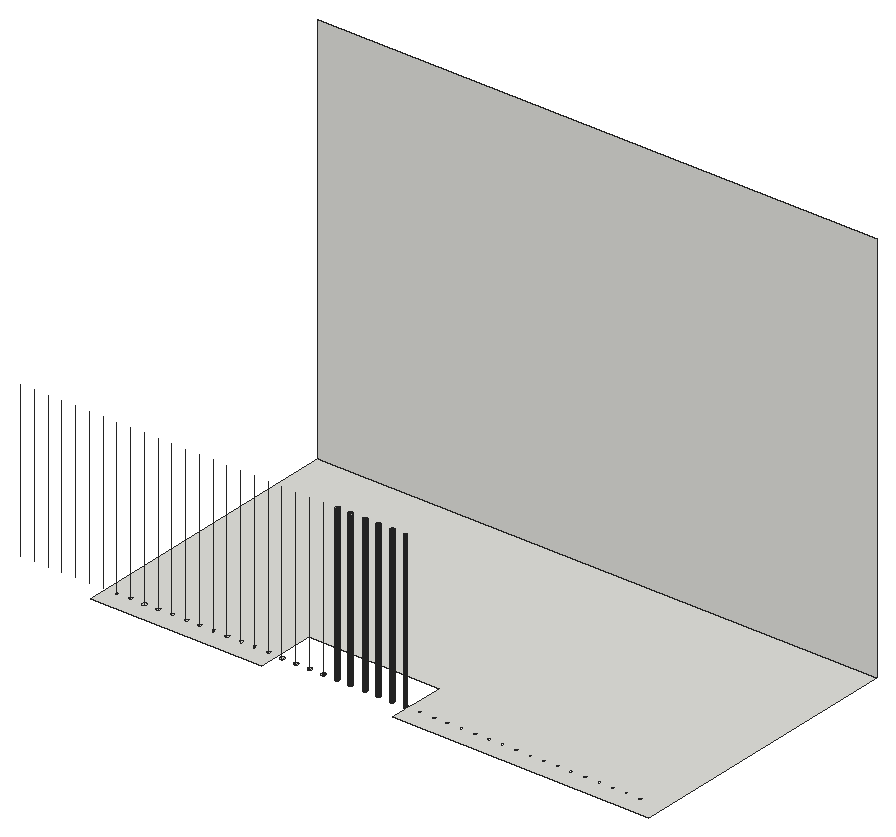
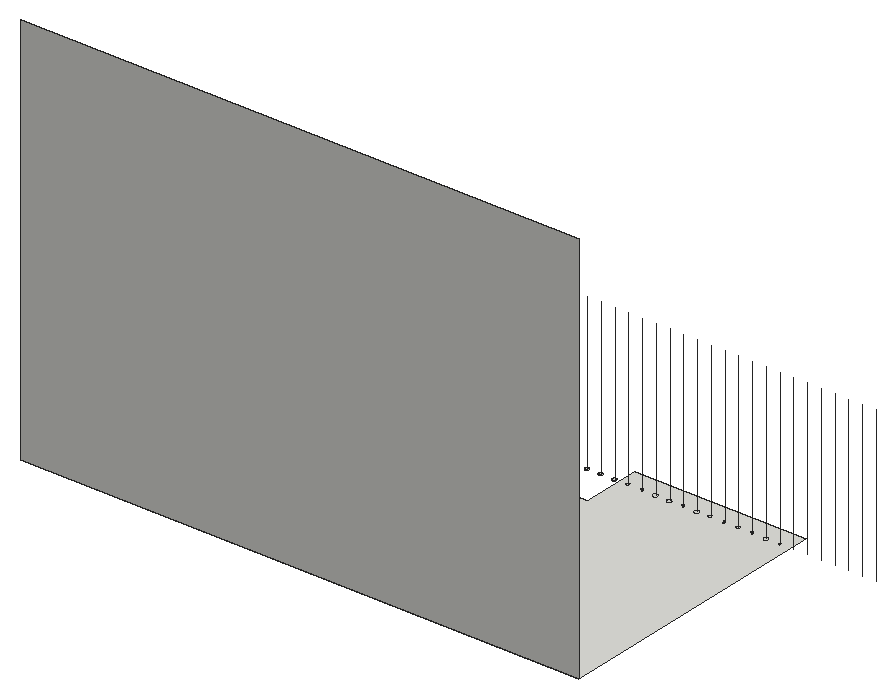
# SketchUp Ruby script. Lengths in inches.
U = 1.inch
M = Sketchup.active_model
def pt(a) = Geom::Point3d.new(a.map { |v| v * U })
def face(e, loops, mat)
  f = e.add_face(loops[0].map { |a| pt(a) })
  loops[1..].each { |l| e.add_face(l.map { |a| pt(a) }).erase! }
  f.material = f.back_material = mat if mat
  f
end
# faces: each face lists its corners as indices into pts; further lists are holes
def faces(e, pts, list, mat = nil) = list.each { |f| face(e, (f[0].is_a?(Array) ? f : [f]).map { |l| l.map { |i| pts[i] } }, mat) }
# xy, xz, yz: faces in a plane at the given z, y or x. An outline is a flat list of corners, or four numbers for a rectangle; further outlines are holes
def ring(l) = l.size == 4 ? [[l[0], l[1]], [l[2], l[1]], [l[2], l[3]], [l[0], l[3]]] : l.each_slice(2).to_a
def flat(e, list, mat, &to3) = list.each { |f| face(e, (f[0].is_a?(Array) ? f : [f]).map { |l| ring(l).map { |u, v| to3.(u, v) } }, mat) }
def xy(e, z, list, mat = nil) = flat(e, list, mat) { |x, y| [x, y, z] }
def xz(e, y, list, mat = nil) = flat(e, list, mat) { |x, z| [x, y, z] }
def yz(e, x, list, mat = nil) = flat(e, list, mat) { |y, z| [x, y, z] }
def lines(e, pts, list) = list.each { |a, b| e.add_line(pt(pts[a]), pt(pts[b])) }
# prism: a flat outline (further loops are holes) pulled along v
def prism(e, loops, v, mat = nil)
  f = face(e, loops, mat); d = Geom::Vector3d.new(v.map { |x| x * U })
  f.pushpull(f.normal.samedirection?(d) ? d.length : -d.length)
end
def box(e, o, s, mat = nil) = prism(e, [[o, [o[0] + s[0], o[1], o[2]], [o[0] + s[0], o[1] + s[1], o[2]], [o[0], o[1] + s[1], o[2]]]], [0, 0, s[2]], mat)
def at(x, y, z, deg = 0) = Geom::Transformation.translation(pt([x, y, z])) * Geom::Transformation.rotation(ORIGIN, Z_AXIS, deg.degrees)
def axes(o, x, y, z) = Geom::Transformation.new([*x, 0, *y, 0, *z, 0, *pt(o).to_a, 1])
def part(name) = M.definitions.add(name)
# library, detail: a bought-in or finely detailed component or shape, given as its bounding box
def library(name, o, s) = part(name).tap { |d| box(d.entities, o, s) }
def detail(e, o, s) = box(e.add_group.entities, o, s)
def put(e, d, t, mat = nil) = e.add_instance(d, t).tap { |i| i.material = mat if mat }
def group(e, t, mat = nil) = e.add_group.tap { |g| g.transformation = t; g.material = mat if mat }.entities
root = M.entities
xy(root,614.8125,[[[290.4375,124.5,363.4375,124.5,363.4375,149.5,419.5625,149.5,419.5625,124.5,528.75,124.5,528.75,246,290.4375,246],[300.98,132.01,300.77,132.04,300.58,132.125,300.41,132.25,300.28,132.42,300.2,132.62,300.17,132.83,300.2,133.04,300.28,133.23,300.41,133.4,300.58,133.53,300.77,133.61,300.98,133.64,301.19,133.61,301.39,133.53,301.56,133.4,301.6875,133.23,301.77,133.04,301.8,132.83,301.77,132.62,301.6875,132.42,301.56,132.25,301.39,132.125,301.19,132.04],[306.92,132.01,306.71,132.04,306.51,132.125,306.35,132.25,306.22,132.42,306.14,132.62,306.11,132.83,306.14,133.04,306.22,133.23,306.35,133.4,306.51,133.53,306.71,133.61,306.92,133.64,307.13,133.61,307.33,133.53,307.49,133.4,307.625,133.23,307.7,133.04,307.73,132.83,307.7,132.62,307.625,132.42,307.49,132.25,307.33,132.125,307.13,132.04],[312.8,132.01,312.58,132.04,312.39,132.125,312.22,132.25,312.09,132.42,312.01,132.62,311.98,132.83,312.01,133.04,312.09,133.23,312.22,133.4,312.39,133.53,312.58,133.61,312.8,133.64,313.01,133.61,313.2,133.53,313.37,133.4,313.5,133.23,313.58,133.04,313.61,132.83,313.58,132.62,313.5,132.42,313.37,132.25,313.2,132.125,313.01,132.04],[318.73,132.01,318.52,132.04,318.33,132.125,318.16,132.25,318.03,132.42,317.95,132.62,317.92,132.83,317.95,133.04,318.03,133.23,318.16,133.4,318.33,133.53,318.52,133.61,318.73,133.64,318.94,133.61,319.14,133.53,319.31,133.4,319.4375,133.23,319.52,133.04,319.55,132.83,319.52,132.62,319.4375,132.42,319.31,132.25,319.14,132.125,318.94,132.04],[324.98,132.01,324.77,132.04,324.58,132.125,324.41,132.25,324.28,132.42,324.2,132.62,324.17,132.83,324.2,133.04,324.28,133.23,324.41,133.4,324.58,133.53,324.77,133.61,324.98,133.64,325.19,133.61,325.39,133.53,325.56,133.4,325.6875,133.23,325.77,133.04,325.8,132.83,325.77,132.62,325.6875,132.42,325.56,132.25,325.39,132.125,325.19,132.04],[330.48,132.01,330.27,132.04,330.08,132.125,329.91,132.25,329.78,132.42,329.7,132.62,329.67,132.83,329.7,133.04,329.78,133.23,329.91,133.4,330.08,133.53,330.27,133.61,330.48,133.64,330.69,133.61,330.89,133.53,331.06,133.4,331.1875,133.23,331.27,133.04,331.3,132.83,331.27,132.62,331.1875,132.42,331.06,132.25,330.89,132.125,330.69,132.04],[336.36,132.04,336.14,132.07,335.95,132.15,335.78,132.28,335.65,132.45,335.57,132.64,335.54,132.85,335.57,133.06,335.65,133.26,335.78,133.43,335.95,133.56,336.14,133.64,336.36,133.67,336.57,133.64,336.76,133.56,336.93,133.43,337.06,133.26,337.14,133.06,337.17,132.85,337.14,132.64,337.06,132.45,336.93,132.28,336.76,132.15,336.57,132.07],[342.23,132.04,342.02,132.07,341.82,132.15,341.66,132.28,341.53,132.45,341.45,132.64,341.42,132.85,341.45,133.06,341.53,133.26,341.66,133.43,341.82,133.56,342.02,133.64,342.23,133.67,342.44,133.64,342.64,133.56,342.8,133.43,342.93,133.26,343.02,133.06,343.04,132.85,343.02,132.64,342.93,132.45,342.8,132.28,342.64,132.15,342.44,132.07],[348.23,132.04,348.02,132.07,347.82,132.15,347.66,132.28,347.53,132.45,347.45,132.64,347.42,132.85,347.45,133.06,347.53,133.26,347.66,133.43,347.82,133.56,348.02,133.64,348.23,133.67,348.44,133.64,348.64,133.56,348.8,133.43,348.93,133.26,349.02,133.06,349.04,132.85,349.02,132.64,348.93,132.45,348.8,132.28,348.64,132.15,348.44,132.07],[353.79,132.04,353.58,132.07,353.39,132.15,353.22,132.28,353.09,132.45,353.01,132.64,352.98,132.85,353.01,133.06,353.09,133.26,353.22,133.43,353.39,133.56,353.58,133.64,353.79,133.67,354,133.64,354.2,133.56,354.37,133.43,354.5,133.26,354.58,133.06,354.61,132.85,354.58,132.64,354.5,132.45,354.37,132.28,354.2,132.15,354,132.07],[359.86,132.04,359.64,132.07,359.45,132.15,359.28,132.28,359.15,132.45,359.07,132.64,359.04,132.85,359.07,133.06,359.15,133.26,359.28,133.43,359.45,133.56,359.64,133.64,359.86,133.67,360.07,133.64,360.26,133.56,360.43,133.43,360.56,133.26,360.64,133.06,360.67,132.85,360.64,132.64,360.56,132.45,360.43,132.28,360.26,132.15,360.07,132.07],[365.67,132.04,365.46,132.07,365.26,132.15,365.09,132.28,364.96,132.45,364.88,132.64,364.86,132.85,364.88,133.06,364.96,133.26,365.09,133.43,365.26,133.56,365.46,133.64,365.67,133.67,365.88,133.64,366.07,133.56,366.24,133.43,366.37,133.26,366.45,133.06,366.48,132.85,366.45,132.64,366.37,132.45,366.24,132.28,366.07,132.15,365.88,132.07],[371.48,132.04,371.27,132.07,371.07,132.15,370.91,132.28,370.78,132.45,370.7,132.64,370.67,132.85,370.7,133.06,370.78,133.26,370.91,133.43,371.07,133.56,371.27,133.64,371.48,133.67,371.69,133.64,371.89,133.56,372.05,133.43,372.18,133.26,372.27,133.06,372.29,132.85,372.27,132.64,372.18,132.45,372.05,132.28,371.89,132.15,371.69,132.07],[377.42,132.04,377.21,132.07,377.01,132.15,376.84,132.28,376.71,132.45,376.63,132.64,376.61,132.85,376.63,133.06,376.71,133.26,376.84,133.43,377.01,133.56,377.21,133.64,377.42,133.67,377.63,133.64,377.82,133.56,377.99,133.43,378.12,133.26,378.2,133.06,378.23,132.85,378.2,132.64,378.12,132.45,377.99,132.28,377.82,132.15,377.63,132.07],[383.23,132.04,383.02,132.07,382.82,132.15,382.66,132.28,382.53,132.45,382.45,132.64,382.42,132.85,382.45,133.06,382.53,133.26,382.66,133.43,382.82,133.56,383.02,133.64,383.23,133.67,383.44,133.64,383.64,133.56,383.8,133.43,383.93,133.26,384.02,133.06,384.04,132.85,384.02,132.64,383.93,132.45,383.8,132.28,383.64,132.15,383.44,132.07],[389.17,132.04,388.96,132.07,388.76,132.15,388.59,132.28,388.46,132.45,388.38,132.64,388.36,132.85,388.38,133.06,388.46,133.26,388.59,133.43,388.76,133.56,388.96,133.64,389.17,133.67,389.38,133.64,389.57,133.56,389.74,133.43,389.87,133.26,389.95,133.06,389.98,132.85,389.95,132.64,389.87,132.45,389.74,132.28,389.57,132.15,389.38,132.07],[394.86,132.04,394.64,132.07,394.45,132.15,394.28,132.28,394.15,132.45,394.07,132.64,394.04,132.85,394.07,133.06,394.15,133.26,394.28,133.43,394.45,133.56,394.64,133.64,394.86,133.67,395.07,133.64,395.26,133.56,395.43,133.43,395.56,133.26,395.64,133.06,395.67,132.85,395.64,132.64,395.56,132.45,395.43,132.28,395.26,132.15,395.07,132.07],[400.92,132.04,400.71,132.07,400.51,132.15,400.34,132.28,400.21,132.45,400.13,132.64,400.11,132.85,400.13,133.06,400.21,133.26,400.34,133.43,400.51,133.56,400.71,133.64,400.92,133.67,401.13,133.64,401.32,133.56,401.49,133.43,401.62,133.26,401.7,133.06,401.73,132.85,401.7,132.64,401.62,132.45,401.49,132.28,401.32,132.15,401.13,132.07],[406.79,132.04,406.58,132.07,406.39,132.15,406.22,132.28,406.09,132.45,406.01,132.64,405.98,132.85,406.01,133.06,406.09,133.26,406.22,133.43,406.39,133.56,406.58,133.64,406.79,133.67,407,133.64,407.2,133.56,407.37,133.43,407.5,133.26,407.58,133.06,407.61,132.85,407.58,132.64,407.5,132.45,407.37,132.28,407.2,132.15,407,132.07],[412.67,132.04,412.46,132.07,412.26,132.15,412.09,132.28,411.96,132.45,411.88,132.64,411.86,132.85,411.88,133.06,411.96,133.26,412.09,133.43,412.26,133.56,412.46,133.64,412.67,133.67,412.88,133.64,413.07,133.56,413.24,133.43,413.37,133.26,413.45,133.06,413.48,132.85,413.45,132.64,413.37,132.45,413.24,132.28,413.07,132.15,412.88,132.07],[418.54,132.04,418.33,132.07,418.14,132.15,417.97,132.28,417.84,132.45,417.76,132.64,417.73,132.85,417.76,133.06,417.84,133.26,417.97,133.43,418.14,133.56,418.33,133.64,418.54,133.67,418.75,133.64,418.95,133.56,419.12,133.43,419.25,133.26,419.33,133.06,419.36,132.85,419.33,132.64,419.25,132.45,419.12,132.28,418.95,132.15,418.75,132.07],[424.36,132.04,424.14,132.07,423.95,132.15,423.78,132.28,423.65,132.45,423.57,132.64,423.54,132.85,423.57,133.06,423.65,133.26,423.78,133.43,423.95,133.56,424.14,133.64,424.36,133.67,424.57,133.64,424.76,133.56,424.93,133.43,425.06,133.26,425.14,133.06,425.17,132.85,425.14,132.64,425.06,132.45,424.93,132.28,424.76,132.15,424.57,132.07],[430.54,132.04,430.33,132.07,430.14,132.15,429.97,132.28,429.84,132.45,429.76,132.64,429.73,132.85,429.76,133.06,429.84,133.26,429.97,133.43,430.14,133.56,430.33,133.64,430.54,133.67,430.75,133.64,430.95,133.56,431.12,133.43,431.25,133.26,431.33,133.06,431.36,132.85,431.33,132.64,431.25,132.45,431.12,132.28,430.95,132.15,430.75,132.07],[436.11,132.04,435.89,132.07,435.7,132.15,435.53,132.28,435.4,132.45,435.32,132.64,435.29,132.85,435.32,133.06,435.4,133.26,435.53,133.43,435.7,133.56,435.89,133.64,436.11,133.67,436.32,133.64,436.51,133.56,436.68,133.43,436.81,133.26,436.89,133.06,436.92,132.85,436.89,132.64,436.81,132.45,436.68,132.28,436.51,132.15,436.32,132.07],[442.11,132.04,441.89,132.07,441.7,132.15,441.53,132.28,441.4,132.45,441.32,132.64,441.29,132.85,441.32,133.06,441.4,133.26,441.53,133.43,441.7,133.56,441.89,133.64,442.11,133.67,442.32,133.64,442.51,133.56,442.68,133.43,442.81,133.26,442.89,133.06,442.92,132.85,442.89,132.64,442.81,132.45,442.68,132.28,442.51,132.15,442.32,132.07],[447.98,132.04,447.77,132.07,447.57,132.15,447.41,132.28,447.28,132.45,447.2,132.64,447.17,132.85,447.2,133.06,447.28,133.26,447.41,133.43,447.57,133.56,447.77,133.64,447.98,133.67,448.19,133.64,448.39,133.56,448.55,133.43,448.68,133.26,448.77,133.06,448.79,132.85,448.77,132.64,448.68,132.45,448.55,132.28,448.39,132.15,448.19,132.07],[453.86,132.04,453.64,132.07,453.45,132.15,453.28,132.28,453.15,132.45,453.07,132.64,453.04,132.85,453.07,133.06,453.15,133.26,453.28,133.43,453.45,133.56,453.64,133.64,453.86,133.67,454.07,133.64,454.26,133.56,454.43,133.43,454.56,133.26,454.64,133.06,454.67,132.85,454.64,132.64,454.56,132.45,454.43,132.28,454.26,132.15,454.07,132.07],[459.48,132.04,459.27,132.07,459.07,132.15,458.91,132.28,458.78,132.45,458.7,132.64,458.67,132.85,458.7,133.06,458.78,133.26,458.91,133.43,459.07,133.56,459.27,133.64,459.48,133.67,459.69,133.64,459.89,133.56,460.05,133.43,460.18,133.26,460.27,133.06,460.29,132.85,460.27,132.64,460.18,132.45,460.05,132.28,459.89,132.15,459.69,132.07],[465.54,132.04,465.33,132.07,465.14,132.15,464.97,132.28,464.84,132.45,464.76,132.64,464.73,132.85,464.76,133.06,464.84,133.26,464.97,133.43,465.14,133.56,465.33,133.64,465.54,133.67,465.75,133.64,465.95,133.56,466.12,133.43,466.25,133.26,466.33,133.06,466.36,132.85,466.33,132.64,466.25,132.45,466.12,132.28,465.95,132.15,465.75,132.07],[471.54,132.04,471.33,132.07,471.14,132.15,470.97,132.28,470.84,132.45,470.76,132.64,470.73,132.85,470.76,133.06,470.84,133.26,470.97,133.43,471.14,133.56,471.33,133.64,471.54,133.67,471.75,133.64,471.95,133.56,472.12,133.43,472.25,133.26,472.33,133.06,472.36,132.85,472.33,132.64,472.25,132.45,472.12,132.28,471.95,132.15,471.75,132.07],[477.23,132.04,477.02,132.07,476.82,132.15,476.66,132.28,476.53,132.45,476.45,132.64,476.42,132.85,476.45,133.06,476.53,133.26,476.66,133.43,476.82,133.56,477.02,133.64,477.23,133.67,477.44,133.64,477.64,133.56,477.8,133.43,477.93,133.26,478.02,133.06,478.04,132.85,478.02,132.64,477.93,132.45,477.8,132.28,477.64,132.15,477.44,132.07],[483.11,132.04,482.89,132.07,482.7,132.15,482.53,132.28,482.4,132.45,482.32,132.64,482.29,132.85,482.32,133.06,482.4,133.26,482.53,133.43,482.7,133.56,482.89,133.64,483.11,133.67,483.32,133.64,483.51,133.56,483.68,133.43,483.81,133.26,483.89,133.06,483.92,132.85,483.89,132.64,483.81,132.45,483.68,132.28,483.51,132.15,483.32,132.07],[488.98,132.04,488.77,132.07,488.57,132.15,488.41,132.28,488.28,132.45,488.2,132.64,488.17,132.85,488.2,133.06,488.28,133.26,488.41,133.43,488.57,133.56,488.77,133.64,488.98,133.67,489.19,133.64,489.39,133.56,489.55,133.43,489.68,133.26,489.77,133.06,489.79,132.85,489.77,132.64,489.68,132.45,489.55,132.28,489.39,132.15,489.19,132.07],[518.54,132.04,518.33,132.07,518.14,132.15,517.97,132.28,517.84,132.45,517.76,132.64,517.73,132.85,517.76,133.06,517.84,133.26,517.97,133.43,518.14,133.56,518.33,133.64,518.54,133.67,518.75,133.64,518.95,133.56,519.12,133.43,519.25,133.26,519.33,133.06,519.36,132.85,519.33,132.64,519.25,132.45,519.12,132.28,518.95,132.15,518.75,132.07],[512.54,132.04,512.33,132.07,512.14,132.15,511.97,132.28,511.84,132.45,511.76,132.64,511.73,132.85,511.76,133.06,511.84,133.26,511.97,133.43,512.14,133.56,512.33,133.64,512.54,133.67,512.75,133.64,512.95,133.56,513.12,133.43,513.25,133.26,513.33,133.06,513.36,132.85,513.33,132.64,513.25,132.45,513.12,132.28,512.95,132.15,512.75,132.07],[506.67,132.04,506.46,132.07,506.26,132.15,506.09,132.28,505.96,132.45,505.88,132.64,505.86,132.85,505.88,133.06,505.96,133.26,506.09,133.43,506.26,133.56,506.46,133.64,506.67,133.67,506.88,133.64,507.07,133.56,507.24,133.43,507.37,133.26,507.45,133.06,507.48,132.85,507.45,132.64,507.37,132.45,507.24,132.28,507.07,132.15,506.88,132.07],[500.86,132.04,500.64,132.07,500.45,132.15,500.28,132.28,500.15,132.45,500.07,132.64,500.04,132.85,500.07,133.06,500.15,133.26,500.28,133.43,500.45,133.56,500.64,133.64,500.86,133.67,501.07,133.64,501.26,133.56,501.43,133.43,501.56,133.26,501.64,133.06,501.67,132.85,501.64,132.64,501.56,132.45,501.43,132.28,501.26,132.15,501.07,132.07],[494.92,132.04,494.71,132.07,494.51,132.15,494.34,132.28,494.21,132.45,494.13,132.64,494.11,132.85,494.13,133.06,494.21,133.26,494.34,133.43,494.51,133.56,494.71,133.64,494.92,133.67,495.13,133.64,495.32,133.56,495.49,133.43,495.62,133.26,495.7,133.06,495.73,132.85,495.7,132.64,495.62,132.45,495.49,132.28,495.32,132.15,495.13,132.07],[294.98,132.01,294.77,132.04,294.58,132.125,294.41,132.25,294.28,132.42,294.2,132.62,294.17,132.83,294.2,133.04,294.28,133.23,294.41,133.4,294.58,133.53,294.77,133.61,294.98,133.64,295.19,133.61,295.39,133.53,295.56,133.4,295.6875,133.23,295.77,133.04,295.8,132.83,295.77,132.62,295.6875,132.42,295.56,132.25,295.39,132.125,295.19,132.04]],[300.98,132.01,300.77,132.04,300.58,132.125,300.41,132.25,300.28,132.42,300.2,132.62,300.17,132.83,300.2,133.04,300.28,133.23,300.41,133.4,300.58,133.53,300.77,133.61,300.98,133.64,301.19,133.61,301.39,133.53,301.56,133.4,301.6875,133.23,301.77,133.04,301.8,132.83,301.77,132.62,301.6875,132.42,301.56,132.25,301.39,132.125,301.19,132.04],[306.92,132.01,306.71,132.04,306.51,132.125,306.35,132.25,306.22,132.42,306.14,132.62,306.11,132.83,306.14,133.04,306.22,133.23,306.35,133.4,306.51,133.53,306.71,133.61,306.92,133.64,307.13,133.61,307.33,133.53,307.49,133.4,307.625,133.23,307.7,133.04,307.73,132.83,307.7,132.62,307.625,132.42,307.49,132.25,307.33,132.125,307.13,132.04],[312.8,132.01,312.58,132.04,312.39,132.125,312.22,132.25,312.09,132.42,312.01,132.62,311.98,132.83,312.01,133.04,312.09,133.23,312.22,133.4,312.39,133.53,312.58,133.61,312.8,133.64,313.01,133.61,313.2,133.53,313.37,133.4,313.5,133.23,313.58,133.04,313.61,132.83,313.58,132.62,313.5,132.42,313.37,132.25,313.2,132.125,313.01,132.04],[318.73,132.01,318.52,132.04,318.33,132.125,318.16,132.25,318.03,132.42,317.95,132.62,317.92,132.83,317.95,133.04,318.03,133.23,318.16,133.4,318.33,133.53,318.52,133.61,318.73,133.64,318.94,133.61,319.14,133.53,319.31,133.4,319.4375,133.23,319.52,133.04,319.55,132.83,319.52,132.62,319.4375,132.42,319.31,132.25,319.14,132.125,318.94,132.04],
  [324.98,132.01,324.77,132.04,324.58,132.125,324.41,132.25,324.28,132.42,324.2,132.62,324.17,132.83,324.2,133.04,324.28,133.23,324.41,133.4,324.58,133.53,324.77,133.61,324.98,133.64,325.19,133.61,325.39,133.53,325.56,133.4,325.6875,133.23,325.77,133.04,325.8,132.83,325.77,132.62,325.6875,132.42,325.56,132.25,325.39,132.125,325.19,132.04],[330.48,132.01,330.27,132.04,330.08,132.125,329.91,132.25,329.78,132.42,329.7,132.62,329.67,132.83,329.7,133.04,329.78,133.23,329.91,133.4,330.08,133.53,330.27,133.61,330.48,133.64,330.69,133.61,330.89,133.53,331.06,133.4,331.1875,133.23,331.27,133.04,331.3,132.83,331.27,132.62,331.1875,132.42,331.06,132.25,330.89,132.125,330.69,132.04],[336.36,132.04,336.14,132.07,335.95,132.15,335.78,132.28,335.65,132.45,335.57,132.64,335.54,132.85,335.57,133.06,335.65,133.26,335.78,133.43,335.95,133.56,336.14,133.64,336.36,133.67,336.57,133.64,336.76,133.56,336.93,133.43,337.06,133.26,337.14,133.06,337.17,132.85,337.14,132.64,337.06,132.45,336.93,132.28,336.76,132.15,336.57,132.07],[342.23,132.04,342.02,132.07,341.82,132.15,341.66,132.28,341.53,132.45,341.45,132.64,341.42,132.85,341.45,133.06,341.53,133.26,341.66,133.43,341.82,133.56,342.02,133.64,342.23,133.67,342.44,133.64,342.64,133.56,342.8,133.43,342.93,133.26,343.02,133.06,343.04,132.85,343.02,132.64,342.93,132.45,342.8,132.28,342.64,132.15,342.44,132.07],[348.23,132.04,348.02,132.07,347.82,132.15,347.66,132.28,347.53,132.45,347.45,132.64,347.42,132.85,347.45,133.06,347.53,133.26,347.66,133.43,347.82,133.56,348.02,133.64,348.23,133.67,348.44,133.64,348.64,133.56,348.8,133.43,348.93,133.26,349.02,133.06,349.04,132.85,349.02,132.64,348.93,132.45,348.8,132.28,348.64,132.15,348.44,132.07],
  [353.79,132.04,353.58,132.07,353.39,132.15,353.22,132.28,353.09,132.45,353.01,132.64,352.98,132.85,353.01,133.06,353.09,133.26,353.22,133.43,353.39,133.56,353.58,133.64,353.79,133.67,354,133.64,354.2,133.56,354.37,133.43,354.5,133.26,354.58,133.06,354.61,132.85,354.58,132.64,354.5,132.45,354.37,132.28,354.2,132.15,354,132.07],[359.86,132.04,359.64,132.07,359.45,132.15,359.28,132.28,359.15,132.45,359.07,132.64,359.04,132.85,359.07,133.06,359.15,133.26,359.28,133.43,359.45,133.56,359.64,133.64,359.86,133.67,360.07,133.64,360.26,133.56,360.43,133.43,360.56,133.26,360.64,133.06,360.67,132.85,360.64,132.64,360.56,132.45,360.43,132.28,360.26,132.15,360.07,132.07],[365.67,132.04,365.46,132.07,365.26,132.15,365.09,132.28,364.96,132.45,364.88,132.64,364.86,132.85,364.88,133.06,364.96,133.26,365.09,133.43,365.26,133.56,365.46,133.64,365.67,133.67,365.88,133.64,366.07,133.56,366.24,133.43,366.37,133.26,366.45,133.06,366.48,132.85,366.45,132.64,366.37,132.45,366.24,132.28,366.07,132.15,365.88,132.07],[371.48,132.04,371.27,132.07,371.07,132.15,370.91,132.28,370.78,132.45,370.7,132.64,370.67,132.85,370.7,133.06,370.78,133.26,370.91,133.43,371.07,133.56,371.27,133.64,371.48,133.67,371.69,133.64,371.89,133.56,372.05,133.43,372.18,133.26,372.27,133.06,372.29,132.85,372.27,132.64,372.18,132.45,372.05,132.28,371.89,132.15,371.69,132.07],[377.42,132.04,377.21,132.07,377.01,132.15,376.84,132.28,376.71,132.45,376.63,132.64,376.61,132.85,376.63,133.06,376.71,133.26,376.84,133.43,377.01,133.56,377.21,133.64,377.42,133.67,377.63,133.64,377.82,133.56,377.99,133.43,378.12,133.26,378.2,133.06,378.23,132.85,378.2,132.64,378.12,132.45,377.99,132.28,377.82,132.15,377.63,132.07],
  [383.23,132.04,383.02,132.07,382.82,132.15,382.66,132.28,382.53,132.45,382.45,132.64,382.42,132.85,382.45,133.06,382.53,133.26,382.66,133.43,382.82,133.56,383.02,133.64,383.23,133.67,383.44,133.64,383.64,133.56,383.8,133.43,383.93,133.26,384.02,133.06,384.04,132.85,384.02,132.64,383.93,132.45,383.8,132.28,383.64,132.15,383.44,132.07],[389.17,132.04,388.96,132.07,388.76,132.15,388.59,132.28,388.46,132.45,388.38,132.64,388.36,132.85,388.38,133.06,388.46,133.26,388.59,133.43,388.76,133.56,388.96,133.64,389.17,133.67,389.38,133.64,389.57,133.56,389.74,133.43,389.87,133.26,389.95,133.06,389.98,132.85,389.95,132.64,389.87,132.45,389.74,132.28,389.57,132.15,389.38,132.07],[394.86,132.04,394.64,132.07,394.45,132.15,394.28,132.28,394.15,132.45,394.07,132.64,394.04,132.85,394.07,133.06,394.15,133.26,394.28,133.43,394.45,133.56,394.64,133.64,394.86,133.67,395.07,133.64,395.26,133.56,395.43,133.43,395.56,133.26,395.64,133.06,395.67,132.85,395.64,132.64,395.56,132.45,395.43,132.28,395.26,132.15,395.07,132.07],[400.92,132.04,400.71,132.07,400.51,132.15,400.34,132.28,400.21,132.45,400.13,132.64,400.11,132.85,400.13,133.06,400.21,133.26,400.34,133.43,400.51,133.56,400.71,133.64,400.92,133.67,401.13,133.64,401.32,133.56,401.49,133.43,401.62,133.26,401.7,133.06,401.73,132.85,401.7,132.64,401.62,132.45,401.49,132.28,401.32,132.15,401.13,132.07],[406.79,132.04,406.58,132.07,406.39,132.15,406.22,132.28,406.09,132.45,406.01,132.64,405.98,132.85,406.01,133.06,406.09,133.26,406.22,133.43,406.39,133.56,406.58,133.64,406.79,133.67,407,133.64,407.2,133.56,407.37,133.43,407.5,133.26,407.58,133.06,407.61,132.85,407.58,132.64,407.5,132.45,407.37,132.28,407.2,132.15,407,132.07],
  [412.67,132.04,412.46,132.07,412.26,132.15,412.09,132.28,411.96,132.45,411.88,132.64,411.86,132.85,411.88,133.06,411.96,133.26,412.09,133.43,412.26,133.56,412.46,133.64,412.67,133.67,412.88,133.64,413.07,133.56,413.24,133.43,413.37,133.26,413.45,133.06,413.48,132.85,413.45,132.64,413.37,132.45,413.24,132.28,413.07,132.15,412.88,132.07]])
xz(root,246,[[290.4375,614.8125,528.75,782.8125]])
p = [[389.17,132.04,614.8125],[389.38,132.07,614.8125],[389.38,132.07,680.58],[389.17,132.04,680.58],[394.64,132.07,614.8125],[394.86,132.04,614.8125],
  [394.86,132.04,680.58],[394.64,132.07,680.58],[395.07,132.07,614.8125],[395.07,132.07,680.58],[400.71,132.07,614.8125],[400.92,132.04,614.8125],
  [400.92,132.04,680.58],[400.71,132.07,680.58],[401.13,132.07,614.8125],[401.13,132.07,680.58],[406.58,132.07,614.8125],[406.79,132.04,614.8125],
  [406.79,132.04,680.58],[406.58,132.07,680.58],[407,132.07,614.8125],[407,132.07,680.58],[412.46,132.07,614.8125],[412.67,132.04,614.8125],
  [412.67,132.04,680.58],[412.46,132.07,680.58],[412.88,132.07,614.8125],[412.88,132.07,680.58],[389.57,132.15,614.8125],[389.57,132.15,680.58],
  [394.45,132.15,614.8125],[394.45,132.15,680.58],[395.26,132.15,614.8125],[395.26,132.15,680.58],[400.51,132.15,614.8125],[400.51,132.15,680.58],
  [401.32,132.15,614.8125],[401.32,132.15,680.58],[406.39,132.15,614.8125],[406.39,132.15,680.58],[407.2,132.15,614.8125],[407.2,132.15,680.58],
  [412.26,132.15,614.8125],[412.26,132.15,680.58],[413.07,132.15,614.8125],[413.07,132.15,680.58],[418.14,132.15,614.8125],[418.33,132.07,614.8125],
  [418.33,132.07,680.58],[418.14,132.15,680.58],[389.74,132.28,614.8125],[389.74,132.28,680.58],[394.28,132.28,614.8125],[394.28,132.28,680.58],
  [395.43,132.28,614.8125],[395.43,132.28,680.58],[400.34,132.28,614.8125],[400.34,132.28,680.58],[401.49,132.28,614.8125],[401.49,132.28,680.58],
  [406.22,132.28,614.8125],[406.22,132.28,680.58],[407.37,132.28,614.8125],[407.37,132.28,680.58],[412.09,132.28,614.8125],[412.09,132.28,680.58],
  [413.24,132.28,614.8125],[413.24,132.28,680.58],[417.97,132.28,614.8125],[417.97,132.28,680.58],[389.87,132.45,614.8125],[389.87,132.45,680.58],
  [394.15,132.45,614.8125],[394.15,132.45,680.58],[395.56,132.45,614.8125],[395.56,132.45,680.58],[400.21,132.45,614.8125],[400.21,132.45,680.58],
  [401.62,132.45,614.8125],[401.62,132.45,680.58],[406.09,132.45,614.8125],[406.09,132.45,680.58],[407.5,132.45,614.8125],[407.5,132.45,680.58],
  [411.96,132.45,614.8125],[411.96,132.45,680.58],[413.37,132.45,614.8125],[413.37,132.45,680.58],[417.84,132.45,614.8125],[417.84,132.45,680.58],
  [389.95,132.64,614.8125],[389.95,132.64,680.58],[394.07,132.64,614.8125],[394.07,132.64,680.58],[395.64,132.64,614.8125],[395.64,132.64,680.58],
  [400.13,132.64,614.8125],[400.13,132.64,680.58],[401.7,132.64,614.8125],[401.7,132.64,680.58],[406.01,132.64,614.8125],[406.01,132.64,680.58],
  [407.58,132.64,614.8125],[407.58,132.64,680.58],[411.88,132.64,614.8125],[411.88,132.64,680.58],[413.45,132.64,614.8125],[413.45,132.64,680.58],
  [417.76,132.64,614.8125],[417.76,132.64,680.58],[388.36,132.85,614.8125],[388.38,132.64,614.8125],[388.38,132.64,680.58],[388.36,132.85,680.58],
  [389.98,132.85,614.8125],[389.98,132.85,680.58],[394.04,132.85,614.8125],[394.04,132.85,680.58],[395.67,132.85,614.8125],[395.67,132.85,680.58],
  [400.11,132.85,614.8125],[400.11,132.85,680.58],[401.73,132.85,614.8125],[401.73,132.85,680.58],[405.98,132.85,614.8125],[405.98,132.85,680.58],
  [407.61,132.85,614.8125],[407.61,132.85,680.58],[411.86,132.85,614.8125],[411.86,132.85,680.58],[413.48,132.85,614.8125],[413.48,132.85,680.58],
  [417.73,132.85,614.8125],[417.73,132.85,680.58],[388.38,133.06,614.8125],[388.38,133.06,680.58],[389.95,133.06,614.8125],[389.95,133.06,680.58],
  [394.07,133.06,614.8125],[394.07,133.06,680.58],[395.64,133.06,614.8125],[395.64,133.06,680.58],[400.13,133.06,614.8125],[400.13,133.06,680.58],
  [401.7,133.06,614.8125],[401.7,133.06,680.58],[406.01,133.06,614.8125],[406.01,133.06,680.58],[407.58,133.06,614.8125],[407.58,133.06,680.58],
  [411.88,133.06,614.8125],[411.88,133.06,680.58],[413.45,133.06,614.8125],[413.45,133.06,680.58],[417.76,133.06,614.8125],[417.76,133.06,680.58],
  [388.46,133.26,614.8125],[388.46,133.26,680.58],[389.87,133.26,614.8125],[389.87,133.26,680.58],[394.15,133.26,614.8125],[394.15,133.26,680.58],
  [395.56,133.26,614.8125],[395.56,133.26,680.58],[400.21,133.26,614.8125],[400.21,133.26,680.58],[401.62,133.26,614.8125],[401.62,133.26,680.58],
  [406.09,133.26,614.8125],[406.09,133.26,680.58],[407.5,133.26,614.8125],[407.5,133.26,680.58],[411.96,133.26,614.8125],[411.96,133.26,680.58],
  [413.37,133.26,614.8125],[413.37,133.26,680.58],[417.84,133.26,614.8125],[417.84,133.26,680.58],[388.59,133.43,614.8125],[388.59,133.43,680.58],
  [389.74,133.43,614.8125],[389.74,133.43,680.58],[394.28,133.43,614.8125],[394.28,133.43,680.58],[395.43,133.43,614.8125],[395.43,133.43,680.58],
  [400.34,133.43,614.8125],[400.34,133.43,680.58],[401.49,133.43,614.8125],[401.49,133.43,680.58],[406.22,133.43,614.8125],[406.22,133.43,680.58],
  [407.37,133.43,614.8125],[407.37,133.43,680.58],[412.09,133.43,614.8125],[412.09,133.43,680.58],[413.24,133.43,614.8125],[413.24,133.43,680.58],
  [417.97,133.43,614.8125],[417.97,133.43,680.58],[388.76,133.56,614.8125],[388.76,133.56,680.58],[389.57,133.56,614.8125],[389.57,133.56,680.58],
  [394.45,133.56,614.8125],[394.45,133.56,680.58],[395.26,133.56,614.8125],[395.26,133.56,680.58],[400.51,133.56,614.8125],[400.51,133.56,680.58],
  [401.32,133.56,614.8125],[401.32,133.56,680.58],[406.39,133.56,614.8125],[406.39,133.56,680.58],[407.2,133.56,614.8125],[407.2,133.56,680.58],
  [412.26,133.56,614.8125],[412.26,133.56,680.58],[413.07,133.56,614.8125],[413.07,133.56,680.58],[418.14,133.56,614.8125],[418.14,133.56,680.58],
  [388.96,133.64,614.8125],[388.96,133.64,680.58],[389.17,133.67,614.8125],[389.17,133.67,680.58],[389.38,133.64,614.8125],[389.38,133.64,680.58],
  [394.64,133.64,614.8125],[394.64,133.64,680.58],[394.86,133.67,614.8125],[394.86,133.67,680.58],[395.07,133.64,614.8125],[395.07,133.64,680.58],
  [400.71,133.64,614.8125],[400.71,133.64,680.58],[400.92,133.67,614.8125],[400.92,133.67,680.58],[401.13,133.64,614.8125],[401.13,133.64,680.58],
  [406.58,133.64,614.8125],[406.58,133.64,680.58],[406.79,133.67,614.8125],[406.79,133.67,680.58],[407,133.64,614.8125],[407,133.64,680.58],
  [412.46,133.64,614.8125],[412.46,133.64,680.58],[412.67,133.67,614.8125],[412.67,133.67,680.58],[412.88,133.64,614.8125],[412.88,133.64,680.58],
  [418.33,133.64,614.8125],[418.33,133.64,680.58],[412.63,132.57,680.58],[412.63,132.57,614.8125],[406.76,132.57,680.58],[406.76,132.57,614.8125],
  [400.88,132.57,680.58],[400.88,132.57,614.8125],[395.01,132.57,680.58],[395.01,132.57,614.8125],[389.13,132.57,680.58],[389.13,132.57,614.8125],
  [383.26,132.57,680.58],[383.26,132.57,614.8125],[377.38,132.57,680.58],[377.38,132.57,614.8125],[371.51,132.57,680.58],[371.51,132.57,614.8125],
  [365.63,132.57,680.58],[365.63,132.57,614.8125],[359.76,132.57,680.58],[359.76,132.57,614.8125],[353.88,132.57,680.58],[353.88,132.57,614.8125],
  [348.01,132.57,680.58],[348.01,132.57,614.8125],[342.13,132.57,680.58],[342.13,132.57,614.8125],[336.26,132.57,680.58],[336.26,132.57,614.8125],
  [330.38,132.57,680.58],[330.38,132.57,614.8125],[324.51,132.57,680.58],[324.51,132.57,614.8125],[318.63,132.57,680.58],[318.63,132.57,614.8125],
  [312.76,132.57,680.58],[312.76,132.57,614.8125],[306.88,132.57,680.58],[306.88,132.57,614.8125],[301.01,132.57,680.58],[301.01,132.57,614.8125],
  [295.13,132.57,680.58],[295.13,132.57,614.8125],[289.26,132.57,680.58],[289.26,132.57,614.8125],[283.38,132.57,680.58],[283.38,132.57,614.8125],
  [277.51,132.57,680.58],[277.51,132.57,614.8125],[271.63,132.57,680.58],[271.63,132.57,614.8125],[265.76,132.57,680.58],[265.76,132.57,614.8125],
  [259.88,132.57,680.58],[259.88,132.57,614.8125],[254.01,132.57,680.58],[254.01,132.57,614.8125]]
faces(root,p,[[0,1,2,3],[4,5,6,7],[5,8,9,6],[10,11,12,13],[11,14,15,12],[16,17,18,19],[17,20,21,18],[22,23,24,25],
  [23,26,27,24],[1,28,29,2],[30,4,7,31],[8,32,33,9],[34,10,13,35],[14,36,37,15],[38,16,19,39],[20,40,41,21],
  [42,22,25,43],[26,44,45,27],[46,47,48,49],[28,50,51,29],[52,30,31,53],[32,54,55,33],[56,34,35,57],[36,58,59,37],
  [60,38,39,61],[40,62,63,41],[64,42,43,65],[44,66,67,45],[68,46,49,69],[50,70,71,51],[72,52,53,73],[54,74,75,55],
  [76,56,57,77],[58,78,79,59],[80,60,61,81],[62,82,83,63],[84,64,65,85],[66,86,87,67],[88,68,69,89],[70,90,91,71],
  [92,72,73,93],[74,94,95,75],[96,76,77,97],[78,98,99,79],[100,80,81,101],[82,102,103,83],[104,84,85,105],[86,106,107,87],
  [108,88,89,109],[110,111,112,113],[90,114,115,91],[116,92,93,117],[94,118,119,95],[120,96,97,121],[98,122,123,99],[124,100,101,125],
  [102,126,127,103],[128,104,105,129],[106,130,131,107],[132,108,109,133],[134,110,113,135],[114,136,137,115],[138,116,117,139],[118,140,141,119],
  [142,120,121,143],[122,144,145,123],[146,124,125,147],[126,148,149,127],[150,128,129,151],[130,152,153,131],[154,132,133,155],[156,134,135,157],
  [136,158,159,137],[160,138,139,161],[140,162,163,141],[164,142,143,165],[144,166,167,145],[168,146,147,169],[148,170,171,149],[172,150,151,173],
  [152,174,175,153],[176,154,155,177],[178,156,157,179],[158,180,181,159],[182,160,161,183],[162,184,185,163],[186,164,165,187],[166,188,189,167],
  [190,168,169,191],[170,192,193,171],[194,172,173,195],[174,196,197,175],[198,176,177,199],[200,178,179,201],[180,202,203,181],[204,182,183,205],
  [184,206,207,185],[208,186,187,209],[188,210,211,189],[212,190,191,213],[192,214,215,193],[216,194,195,217],[196,218,219,197],[220,198,199,221],
  [222,200,201,223],[224,222,223,225],[226,224,225,227],[202,226,227,203],[228,204,205,229],[230,228,229,231],[232,230,231,233],[206,232,233,207],
  [234,208,209,235],[236,234,235,237],[238,236,237,239],[210,238,239,211],[240,212,213,241],[242,240,241,243],[244,242,243,245],[214,244,245,215],
  [246,216,217,247],[248,246,247,249],[250,248,249,251],[218,250,251,219],[252,220,221,253]])
lines(root,p,[[254,255],[256,257],[258,259],[260,261],[262,263],[264,265],[266,267],[268,269],[270,271],[272,273],[274,275],[276,277],
  [278,279],[280,281],[282,283],[284,285],[286,287],[288,289],[290,291],[292,293],[294,295],[296,297],[298,299],[300,301],
  [302,303],[304,305],[306,307],[308,309]])
